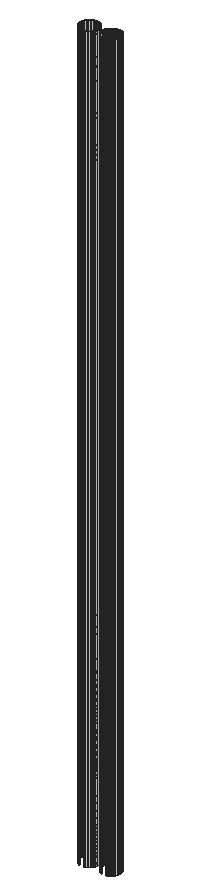
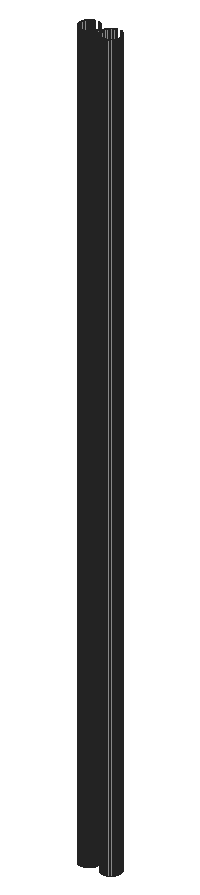
# SketchUp Ruby script. Lengths in inches.
U = 1.inch
M = Sketchup.active_model
def pt(a) = Geom::Point3d.new(a.map { |v| v * U })
def face(e, loops, mat)
  f = e.add_face(loops[0].map { |a| pt(a) })
  loops[1..].each { |l| e.add_face(l.map { |a| pt(a) }).erase! }
  f.material = f.back_material = mat if mat
  f
end
# faces: each face lists its corners as indices into pts; further lists are holes
def faces(e, pts, list, mat = nil) = list.each { |f| face(e, (f[0].is_a?(Array) ? f : [f]).map { |l| l.map { |i| pts[i] } }, mat) }
# xy, xz, yz: faces in a plane at the given z, y or x. An outline is a flat list of corners, or four numbers for a rectangle; further outlines are holes
def ring(l) = l.size == 4 ? [[l[0], l[1]], [l[2], l[1]], [l[2], l[3]], [l[0], l[3]]] : l.each_slice(2).to_a
def flat(e, list, mat, &to3) = list.each { |f| face(e, (f[0].is_a?(Array) ? f : [f]).map { |l| ring(l).map { |u, v| to3.(u, v) } }, mat) }
def xy(e, z, list, mat = nil) = flat(e, list, mat) { |x, y| [x, y, z] }
def xz(e, y, list, mat = nil) = flat(e, list, mat) { |x, z| [x, y, z] }
def yz(e, x, list, mat = nil) = flat(e, list, mat) { |y, z| [x, y, z] }
def lines(e, pts, list) = list.each { |a, b| e.add_line(pt(pts[a]), pt(pts[b])) }
# prism: a flat outline (further loops are holes) pulled along v
def prism(e, loops, v, mat = nil)
  f = face(e, loops, mat); d = Geom::Vector3d.new(v.map { |x| x * U })
  f.pushpull(f.normal.samedirection?(d) ? d.length : -d.length)
end
def box(e, o, s, mat = nil) = prism(e, [[o, [o[0] + s[0], o[1], o[2]], [o[0] + s[0], o[1] + s[1], o[2]], [o[0], o[1] + s[1], o[2]]]], [0, 0, s[2]], mat)
def at(x, y, z, deg = 0) = Geom::Transformation.translation(pt([x, y, z])) * Geom::Transformation.rotation(ORIGIN, Z_AXIS, deg.degrees)
def axes(o, x, y, z) = Geom::Transformation.new([*x, 0, *y, 0, *z, 0, *pt(o).to_a, 1])
def part(name) = M.definitions.add(name)
# library, detail: a bought-in or finely detailed component or shape, given as its bounding box
def library(name, o, s) = part(name).tap { |d| box(d.entities, o, s) }
def detail(e, o, s) = box(e.add_group.entities, o, s)
def put(e, d, t, mat = nil) = e.add_instance(d, t).tap { |i| i.material = mat if mat }
def group(e, t, mat = nil) = e.add_group.tap { |g| g.transformation = t; g.material = mat if mat }.entities
root = M.entities
M.materials.add("M01_Silver_Fog").color = [224, 224, 224]
xz(root,479.82,[[225.02,270,225.11,383.24],[228.33,270,228.42,383.24]],"M01_Silver_Fog")
yz(root,223.76,[[478.29,270,478.38,383.24],[478.38,270,478.47,383.24],[478.47,270,478.55,383.24]],"M01_Silver_Fog")
yz(root,226.55,[[478.3,270,478.39,383.24],[478.39,270,478.47,383.24],[478.47,270,478.5625,383.24]],"M01_Silver_Fog")
yz(root,227.07,[[478.29,270,478.38,383.24],[478.38,270,478.47,383.24],[478.47,270,478.55,383.24]],"M01_Silver_Fog")
yz(root,229.87,[[478.39,270,478.47,383.24]],"M01_Silver_Fog")
p = [[225.38,477.04,270],[225.46,477.06,270],[225.46,477.06,383.24],[225.38,477.04,383.24],[228.69,477.04,270],[228.78,477.06,270],
  [228.78,477.06,383.24],[228.69,477.04,383.24],[224.52,477.18,270],[224.6,477.14,270],[224.6,477.14,383.24],[224.52,477.18,383.24],
  [224.68,477.11,270],[224.68,477.11,383.24],[224.77,477.08,270],[224.77,477.08,383.24],[224.85,477.06,270],[224.85,477.06,383.24],
  [225.55,477.08,270],[225.55,477.08,383.24],[225.63,477.11,270],[225.63,477.11,383.24],[225.71,477.14,270],[225.71,477.14,383.24],
  [225.79,477.18,270],[225.79,477.18,383.24],[227.84,477.18,270],[227.91,477.14,270],[227.91,477.14,383.24],[227.84,477.18,383.24],
  [228,477.11,270],[228,477.11,383.24],[228.08,477.08,270],[228.08,477.08,383.24],[228.17,477.06,270],[228.17,477.06,383.24],
  [228.86,477.08,270],[228.86,477.08,383.24],[228.95,477.11,270],[228.95,477.11,383.24],[229.03,477.14,270],[229.03,477.14,383.24],
  [229.11,477.18,270],[229.11,477.18,383.24],[224.45,477.22,270],[224.45,477.22,383.24],[224.37,477.27,270],[224.37,477.27,383.24],
  [225.87,477.22,270],[225.87,477.22,383.24],[225.95,477.27,270],[225.95,477.27,383.24],[227.68,477.27,270],[227.76,477.22,270],
  [227.76,477.22,383.24],[227.68,477.27,383.24],[229.18,477.22,270],[229.18,477.22,383.24],[229.26,477.27,270],[229.26,477.27,383.24],
  [224.23,477.37,270],[224.3,477.32,270],[224.3,477.32,383.24],[224.23,477.37,383.24],[226.02,477.32,270],[226.02,477.32,383.24],
  [226.08,477.38,270],[226.08,477.38,383.24],[227.54,477.37,270],[227.61,477.32,270],[227.61,477.32,383.24],[227.54,477.37,383.24],
  [229.33,477.32,270],[229.33,477.32,383.24],[229.4,477.38,270],[229.4,477.38,383.24],[224.11,477.5,270],[224.17,477.43,270],
  [224.17,477.43,383.24],[224.11,477.5,383.24],[226.15,477.4375,270],[226.15,477.4375,383.24],[226.21,477.5,270],[226.21,477.5,383.24],
  [227.42,477.5,270],[227.48,477.43,270],[227.48,477.43,383.24],[227.42,477.5,383.24],[229.46,477.4375,270],[229.46,477.4375,383.24],
  [229.52,477.5,270],[229.52,477.5,383.24],[224.05,477.56,270],[224.05,477.56,383.24],[226.26,477.57,270],[226.26,477.57,383.24],
  [227.36,477.56,270],[227.36,477.56,383.24],[229.58,477.57,270],[229.58,477.57,383.24],[224,477.64,270],[224,477.64,383.24],
  [223.95,477.71,270],[223.95,477.71,383.24],[226.32,477.64,270],[226.32,477.64,383.24],[226.36,477.72,270],[226.36,477.72,383.24],
  [227.3125,477.64,270],[227.3125,477.64,383.24],[227.26,477.71,270],[227.26,477.71,383.24],[229.63,477.64,270],[229.63,477.64,383.24],
  [229.67,477.72,270],[229.67,477.72,383.24],[223.91,477.79,270],[223.91,477.79,383.24],[226.4,477.79,270],[226.4,477.79,383.24],
  [227.22,477.79,270],[227.22,477.79,383.24],[229.72,477.79,270],[229.72,477.79,383.24],[223.87,477.87,270],[223.87,477.87,383.24],
  [226.44,477.875,270],[226.44,477.875,383.24],[227.18,477.87,270],[227.18,477.87,383.24],[229.75,477.875,270],[229.75,477.875,383.24],
  [223.84,477.95,270],[223.84,477.95,383.24],[223.8125,478.03,270],[223.8125,478.03,383.24],[226.47,477.96,270],[226.47,477.96,383.24],
  [227.125,478.03,270],[227.15,477.95,270],[227.15,477.95,383.24],[227.125,478.03,383.24],[229.79,477.96,270],[229.79,477.96,383.24],
  [223.79,478.12,270],[223.79,478.12,383.24],[226.5,478.04,270],[226.5,478.04,383.24],[226.52,478.125,270],[226.52,478.125,383.24],
  [227.1,478.12,270],[227.1,478.12,383.24],[229.8125,478.04,270],[229.8125,478.04,383.24],[229.83,478.125,270],[229.83,478.125,383.24],
  [223.77,478.2,270],[223.77,478.2,383.24],[226.54,478.21,270],[226.54,478.21,383.24],[227.09,478.2,270],[227.09,478.2,383.24],
  [229.85,478.21,270],[229.85,478.21,383.24],[223.76,478.29,270],[223.76,478.29,383.24],[226.55,478.3,270],[226.55,478.3,383.24],
  [227.07,478.29,270],[227.07,478.29,383.24],[229.86,478.3,270],[229.86,478.3,383.24],[229.87,478.39,270],[229.87,478.39,383.24],
  [229.87,478.47,270],[229.86,478.5625,270],[229.86,478.5625,383.24],[229.87,478.47,383.24],[223.77,478.64,270],[223.76,478.55,270],
  [223.76,478.55,383.24],[223.77,478.64,383.24],[223.79,478.73,270],[223.79,478.73,383.24],[226.55,478.5625,270],[226.54,478.65,270],
  [226.54,478.65,383.24],[226.55,478.5625,383.24],[226.52,478.74,270],[226.52,478.74,383.24],[227.08,478.64,270],[227.07,478.55,270],
  [227.07,478.55,383.24],[227.08,478.64,383.24],[227.1,478.73,270],[227.1,478.73,383.24],[229.85,478.65,270],[229.85,478.65,383.24],
  [229.83,478.74,270],[229.83,478.74,383.24],[223.81,478.8125,270],[223.81,478.8125,383.24],[226.5,478.82,270],[226.5,478.82,383.24],
  [227.12,478.8125,270],[227.12,478.8125,383.24],[229.81,478.82,270],[229.81,478.82,383.24],[223.84,478.9,270],[223.84,478.9,383.24],
  [226.47,478.9,270],[226.47,478.9,383.24],[227.15,478.9,270],[227.15,478.9,383.24],[229.78,478.9,270],[229.78,478.9,383.24],
  [223.87,478.98,270],[223.87,478.98,383.24],[226.4375,478.99,270],[226.4375,478.99,383.24],[227.18,478.98,270],[227.18,478.98,383.24],
  [229.75,478.99,270],[229.75,478.99,383.24],[223.91,479.06,270],[223.91,479.06,383.24],[226.4,479.07,270],[226.4,479.07,383.24],
  [227.22,479.06,270],[227.22,479.06,383.24],[229.71,479.07,270],[229.71,479.07,383.24],[223.95,479.13,270],[223.95,479.13,383.24],
  [223.99,479.21,270],[223.99,479.21,383.24],[226.36,479.14,270],[226.3125,479.22,270],[226.3125,479.22,383.24],[226.36,479.14,383.24],
  [227.26,479.13,270],[227.26,479.13,383.24],[227.31,479.21,270],[227.31,479.21,383.24],[229.67,479.14,270],[229.62,479.22,270],
  [229.62,479.22,383.24],[229.67,479.14,383.24],[224.05,479.28,270],[224.05,479.28,383.24],[226.26,479.29,270],[226.26,479.29,383.24],
  [227.36,479.28,270],[227.36,479.28,383.24],[229.57,479.29,270],[229.57,479.29,383.24],[224.1,479.35,270],[224.1,479.35,383.24],
  [224.16,479.41,270],[224.16,479.41,383.24],[226.2,479.35,270],[226.2,479.35,383.24],[227.41,479.35,270],[227.41,479.35,383.24],
  [227.47,479.41,270],[227.47,479.41,383.24],[229.51,479.35,270],[229.51,479.35,383.24],[224.23,479.47,270],[224.23,479.47,383.24],
  [226.14,479.42,270],[226.14,479.42,383.24],[226.08,479.48,270],[226.08,479.48,383.24],[227.54,479.47,270],[227.54,479.47,383.24],
  [229.45,479.42,270],[229.39,479.48,270],[229.39,479.48,383.24],[229.45,479.42,383.24],[224.29,479.53,270],[224.29,479.53,383.24],
  [224.36,479.58,270],[224.36,479.58,383.24],[226.01,479.53,270],[225.9375,479.59,270],[225.9375,479.59,383.24],[226.01,479.53,383.24],
  [227.61,479.53,270],[227.61,479.53,383.24],[227.68,479.58,270],[227.68,479.58,383.24],[229.32,479.53,270],[229.32,479.53,383.24],
  [229.25,479.59,270],[229.25,479.59,383.24],[224.4375,479.63,270],[224.4375,479.63,383.24],[224.52,479.67,270],[224.52,479.67,383.24],
  [225.86,479.63,270],[225.79,479.68,270],[225.79,479.68,383.24],[225.86,479.63,383.24],[227.75,479.63,270],[227.75,479.63,383.24],
  [227.83,479.67,270],[227.83,479.67,383.24],[229.18,479.63,270],[229.1,479.68,270],[229.1,479.68,383.24],[229.18,479.63,383.24],
  [224.6,479.71,270],[224.6,479.71,383.24],[224.68,479.74,270],[224.68,479.74,383.24],[224.76,479.77,270],[224.76,479.77,383.24],
  [225.625,479.74,270],[225.54,479.77,270],[225.54,479.77,383.24],[225.625,479.74,383.24],[225.71,479.71,270],[225.71,479.71,383.24],
  [227.91,479.71,270],[227.91,479.71,383.24],[227.99,479.74,270],[227.99,479.74,383.24],[228.07,479.77,270],[228.07,479.77,383.24],
  [229.02,479.71,270],[228.9375,479.74,270],[228.9375,479.74,383.24],[229.02,479.71,383.24],[228.85,479.77,270],[228.85,479.77,383.24],
  [224.85,479.79,270],[224.85,479.79,383.24],[224.93,479.81,270],[224.93,479.81,383.24],[225.02,479.82,270],[225.02,479.82,383.24],
  [225.19,479.83,270],[225.11,479.82,270],[225.11,479.82,383.24],[225.19,479.83,383.24],[225.28,479.82,270],[225.28,479.82,383.24],
  [225.37,479.81,270],[225.37,479.81,383.24],[225.46,479.79,270],[225.46,479.79,383.24],[228.16,479.79,270],[228.16,479.79,383.24],
  [228.24,479.81,270],[228.24,479.81,383.24],[228.33,479.82,270],[228.33,479.82,383.24],[228.51,479.83,270],[228.42,479.82,270],
  [228.42,479.82,383.24],[228.51,479.83,383.24],[228.59,479.82,270],[228.59,479.82,383.24],[228.68,479.81,270],[228.68,479.81,383.24],
  [228.77,479.79,270],[228.77,479.79,383.24]]
faces(root,p,[[0,1,2,3],[4,5,6,7],[8,9,10,11],[9,12,13,10],[12,14,15,13],[14,16,17,15],[1,18,19,2],[18,20,21,19],
  [20,22,23,21],[22,24,25,23],[26,27,28,29],[27,30,31,28],[30,32,33,31],[32,34,35,33],[5,36,37,6],[36,38,39,37],
  [38,40,41,39],[40,42,43,41],[44,8,11,45],[46,44,45,47],[24,48,49,25],[48,50,51,49],[52,53,54,55],[53,26,29,54],
  [42,56,57,43],[56,58,59,57],[60,61,62,63],[61,46,47,62],[50,64,65,51],[64,66,67,65],[68,69,70,71],[69,52,55,70],
  [58,72,73,59],[72,74,75,73],[76,77,78,79],[77,60,63,78],[66,80,81,67],[80,82,83,81],[84,85,86,87],[85,68,71,86],
  [74,88,89,75],[88,90,91,89],[92,76,79,93],[82,94,95,83],[96,84,87,97],[90,98,99,91],[100,92,93,101],[102,100,101,103],
  [94,104,105,95],[104,106,107,105],[108,96,97,109],[110,108,109,111],[98,112,113,99],[112,114,115,113],[116,102,103,117],[106,118,119,107],
  [120,110,111,121],[114,122,123,115],[124,116,117,125],[118,126,127,119],[128,120,121,129],[122,130,131,123],[132,124,125,133],[134,132,133,135],
  [126,136,137,127],[138,139,140,141],[139,128,129,140],[130,142,143,131],[144,134,135,145],[136,146,147,137],[146,148,149,147],[150,138,141,151],
  [142,152,153,143],[152,154,155,153],[156,144,145,157],[148,158,159,149],[160,150,151,161],[154,162,163,155],[164,156,157,165],[158,166,167,159],
  [168,160,161,169],[162,170,171,163],[170,172,173,171],[174,175,176,177],[178,179,180,181],[182,178,181,183],[184,185,186,187],[185,188,189,186],
  [190,191,192,193],[194,190,193,195],[175,196,197,176],[196,198,199,197],[200,182,183,201],[188,202,203,189],[204,194,195,205],[198,206,207,199],
  [208,200,201,209],[202,210,211,203],[212,204,205,213],[206,214,215,207],[216,208,209,217],[210,218,219,211],[220,212,213,221],[214,222,223,215],
  [224,216,217,225],[218,226,227,219],[228,220,221,229],[222,230,231,223],[232,224,225,233],[234,232,233,235],[236,237,238,239],[226,236,239,227],
  [240,228,229,241],[242,240,241,243],[244,245,246,247],[230,244,247,231],[248,234,235,249],[237,250,251,238],[252,242,243,253],[245,254,255,246],
  [256,248,249,257],[258,256,257,259],[250,260,261,251],[262,252,253,263],[264,262,263,265],[254,266,267,255],[268,258,259,269],[260,270,271,261],
  [270,272,273,271],[274,264,265,275],[276,277,278,279],[266,276,279,267],[280,268,269,281],[282,280,281,283],[284,285,286,287],[272,284,287,273],
  [288,274,275,289],[290,288,289,291],[277,292,293,278],[292,294,295,293],[296,282,283,297],[298,296,297,299],[300,301,302,303],[285,300,303,286],
  [304,290,291,305],[306,304,305,307],[308,309,310,311],[294,308,311,295],[312,298,299,313],[314,312,313,315],[316,314,315,317],[318,319,320,321],
  [322,318,321,323],[301,322,323,302],[324,306,307,325],[326,324,325,327],[328,326,327,329],[330,331,332,333],[331,334,335,332],[309,330,333,310],
  [336,316,317,337],[338,336,337,339],[340,338,339,341],[342,343,344,345],[346,342,345,347],[348,346,347,349],[350,348,349,351],[319,350,351,320],
  [352,328,329,353],[354,352,353,355],[356,354,355,357],[358,359,360,361],[362,358,361,363],[364,362,363,365],[366,364,365,367],[334,366,367,335]],"M01_Silver_Fog")
